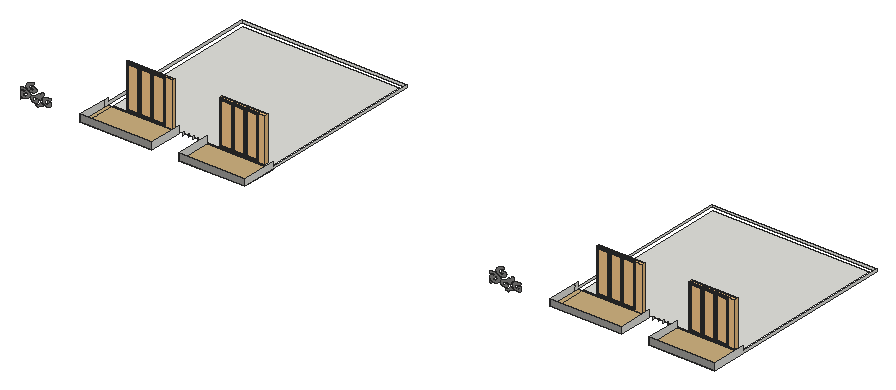
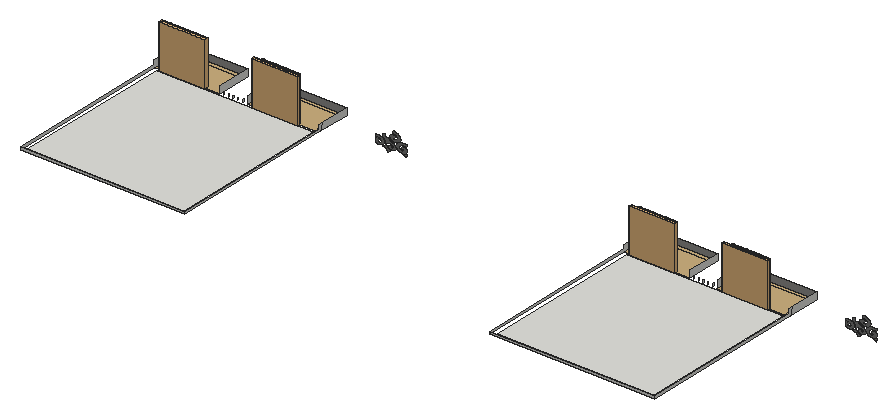
# SketchUp Ruby script. Lengths in inches.
U = 1.inch
M = Sketchup.active_model
def pt(a) = Geom::Point3d.new(a.map { |v| v * U })
def face(e, loops, mat)
  f = e.add_face(loops[0].map { |a| pt(a) })
  loops[1..].each { |l| e.add_face(l.map { |a| pt(a) }).erase! }
  f.material = f.back_material = mat if mat
  f
end
# faces: each face lists its corners as indices into pts; further lists are holes
def faces(e, pts, list, mat = nil) = list.each { |f| face(e, (f[0].is_a?(Array) ? f : [f]).map { |l| l.map { |i| pts[i] } }, mat) }
# xy, xz, yz: faces in a plane at the given z, y or x. An outline is a flat list of corners, or four numbers for a rectangle; further outlines are holes
def ring(l) = l.size == 4 ? [[l[0], l[1]], [l[2], l[1]], [l[2], l[3]], [l[0], l[3]]] : l.each_slice(2).to_a
def flat(e, list, mat, &to3) = list.each { |f| face(e, (f[0].is_a?(Array) ? f : [f]).map { |l| ring(l).map { |u, v| to3.(u, v) } }, mat) }
def xy(e, z, list, mat = nil) = flat(e, list, mat) { |x, y| [x, y, z] }
def xz(e, y, list, mat = nil) = flat(e, list, mat) { |x, z| [x, y, z] }
def yz(e, x, list, mat = nil) = flat(e, list, mat) { |y, z| [x, y, z] }
def lines(e, pts, list) = list.each { |a, b| e.add_line(pt(pts[a]), pt(pts[b])) }
# prism: a flat outline (further loops are holes) pulled along v
def prism(e, loops, v, mat = nil)
  f = face(e, loops, mat); d = Geom::Vector3d.new(v.map { |x| x * U })
  f.pushpull(f.normal.samedirection?(d) ? d.length : -d.length)
end
def box(e, o, s, mat = nil) = prism(e, [[o, [o[0] + s[0], o[1], o[2]], [o[0] + s[0], o[1] + s[1], o[2]], [o[0], o[1] + s[1], o[2]]]], [0, 0, s[2]], mat)
def at(x, y, z, deg = 0) = Geom::Transformation.translation(pt([x, y, z])) * Geom::Transformation.rotation(ORIGIN, Z_AXIS, deg.degrees)
def axes(o, x, y, z) = Geom::Transformation.new([*x, 0, *y, 0, *z, 0, *pt(o).to_a, 1])
def part(name) = M.definitions.add(name)
# library, detail: a bought-in or finely detailed component or shape, given as its bounding box
def library(name, o, s) = part(name).tap { |d| box(d.entities, o, s) }
def detail(e, o, s) = box(e.add_group.entities, o, s)
def put(e, d, t, mat = nil) = e.add_instance(d, t).tap { |i| i.material = mat if mat }
def group(e, t, mat = nil) = e.add_group.tap { |g| g.transformation = t; g.material = mat if mat }.entities
root = M.entities
M.materials.add("Wine2").color = [0, 0, 0]
M.materials["Wine2"].alpha = 0
M.materials.add("[0043_SaddleBrown]4").color = [124, 123, 122]
M.materials.add("[0130_Gainsboro]").color = [39, 45, 50]
M.materials.add("[Granite Light Gray]").color = [149, 148, 144]
M.materials.add("[Wood Floor Light]").color = [204, 176, 127]
c1 = part("Framed glazing panel")
xy(c1.entities,0,[[0,-0.98,43.07,0],[0,0,43.07,1.4]],"[0130_Gainsboro]")
xy(c1.entities,0.3,[[0.3,-1.43,42.77,-0.98]],"[0130_Gainsboro]")
xy(c1.entities,2.95,[[2.95,-1.43,40.12,-0.63],[2.95,-0.63,40.12,0],[2.95,0,40.12,0.64],[2.95,0.64,40.12,1.4]],"[0130_Gainsboro]")
xy(c1.entities,3.54,[[3.54,-0.63,39.53,0],[3.54,0,39.53,0.64]],"[0130_Gainsboro]")
xy(c1.entities,111.8125,[[3.54,-0.63,39.53,0],[3.54,0,39.53,0.64]],"[0130_Gainsboro]")
xy(c1.entities,112.4,[[2.95,-1.43,40.12,-0.63],[2.95,-0.63,40.12,0],[2.95,0,40.12,0.64],[2.95,0.64,40.12,1.4]],"[0130_Gainsboro]")
xy(c1.entities,115.05,[[0.3,-1.43,42.77,-0.98]],"[0130_Gainsboro]")
xy(c1.entities,115.35,[[0,-0.98,43.07,0],[0,0,43.07,1.4]],"[0130_Gainsboro]")
xz(c1.entities,-1.43,[[[0.3,0.3,42.77,115.05],[2.95,2.95,40.12,112.4]]],"[0130_Gainsboro]")
xz(c1.entities,-0.98,[[[0,0,43.07,115.35],[0.3,0.3,42.77,115.05]]],"[0130_Gainsboro]")
xz(c1.entities,-0.63,[[[2.95,2.95,40.12,112.4],[3.54,3.54,39.53,111.8125]]],"[0130_Gainsboro]")
xz(c1.entities,0,[[3.54,3.54,39.53,111.8125]],"Wine2")
xz(c1.entities,0,[[[0,0,43.07,115.35],[2.95,2.95,40.12,112.4]],[[2.95,2.95,40.12,112.4],[3.54,3.54,39.53,111.8125]]],"[0130_Gainsboro]")
xz(c1.entities,0.64,[[[2.95,2.95,40.12,112.4],[3.54,3.54,39.53,111.8125]]],"[0130_Gainsboro]")
xz(c1.entities,1.4,[[[0,0,43.07,115.35],[2.95,2.95,40.12,112.4]]],"[0130_Gainsboro]")
yz(c1.entities,0,[[-0.98,0,0,115.35],[0,0,1.4,115.35]],"[0130_Gainsboro]")
yz(c1.entities,0.3,[[-1.43,0.3,-0.98,115.05]],"[0130_Gainsboro]")
yz(c1.entities,2.95,[[-1.43,2.95,-0.63,112.4],[-0.63,2.95,0,112.4],[0,2.95,0.64,112.4],[0.64,2.95,1.4,112.4]],"[0130_Gainsboro]")
yz(c1.entities,3.54,[[-0.63,3.54,0,111.8125],[0,3.54,0.64,111.8125]],"[0130_Gainsboro]")
yz(c1.entities,39.53,[[-0.63,3.54,0,111.8125],[0,3.54,0.64,111.8125]],"[0130_Gainsboro]")
yz(c1.entities,40.12,[[-1.43,2.95,-0.63,112.4],[-0.63,2.95,0,112.4],[0,2.95,0.64,112.4],[0.64,2.95,1.4,112.4]],"[0130_Gainsboro]")
yz(c1.entities,42.77,[[-1.43,0.3,-0.98,115.05]],"[0130_Gainsboro]")
yz(c1.entities,43.07,[[-0.98,0,0,115.35],[0,0,1.4,115.35]],"[0130_Gainsboro]")
c2 = part("Glazing assembly")
put(c2.entities,c1,axes([90.57,1.43,0],[1.05148,0,0],[0,1,0],[0,0,1]))
put(c2.entities,c1,axes([0,1.43,0],[1.05148,0,0],[0,1,0],[0,0,1]))
put(c2.entities,c1,axes([45.29,1.43,0],[1.05148,0,0],[0,1,0],[0,0,1]))
c3 = library("Curtains",[0,0,0],[121.73,8.19,117.22])
xy(root,514.875,[[3103.26,651.03,3204.51,657.03],[3351.01,651.03,3452.26,657.03],[4353.89,651.03,4455.14,657.03],[4601.63,651.03,4702.88,657.03]])
xy(root,520.4375,[[3064.33,657.03,3480.11,1085.17],[4314.96,657.03,4730.74,1085.17]])
xy(root,520.4375,[[3053.01,559.875,3243.69,570.83],[3316.14,559.875,3491.44,570.83],[4303.63,559.875,4494.32,570.83],[4566.77,559.875,4742.06,570.83],[3053.01,570.83,3064.33,651.03],
  [3064.33,570.83,3243.69,651.03],[3316.14,570.83,3480.11,651.03],[3480.11,570.83,3491.44,651.03],[4303.63,570.83,4314.96,651.03],[4314.96,570.83,4494.32,651.03],
  [4566.77,570.83,4730.74,651.03],[4730.74,570.83,4742.06,651.03]],"[Wood Floor Light]")
xz(root,559.875,[[3053.01,520.4375,3243.69,538.1875],[3316.14,520.4375,3491.44,538.1875],[4303.63,520.4375,4494.32,538.1875],[4566.77,520.4375,4742.06,538.1875]],"[Granite Light Gray]")
xz(root,589.17,[[2918.13,494.52,2917.65,494.86,2917.14,495.2,2916.62,495.53,2916.08,495.84,2915.52,496.14,2914.94,496.43,2914.34,496.71,2913.73,496.97,2913.11,497.21,2912.47,497.45,2911.81,497.67,2911.14,497.87,2912.71,498.36,2914.21,498.91,2915.64,499.53,2917,500.21,2918.28,500.95,2919.47,501.74,2920.5625,502.59,2921.55,503.48,2922.44,504.4,2923.22,505.37,2923.88,506.37,2924.43,507.39,2924.98,507,2925.54,506.61,2926.11,506.23,2926.69,505.86,2927.29,505.49,2927.89,505.13,2928.5,504.77,2929.12,504.42,2930.38,503.74,2931.03,503.41,2931.6875,503.08,2930.03,502.8125,2928.42,502.44,2926.875,501.98,2925.41,501.42,2924.05,500.78,2922.79,500.0625,2921.65,499.27,2920.65,498.42,2919.79,497.5,2919.08,496.54,2918.52,495.54],[4168.75,494.52,4168.27,494.86,4167.77,495.2,4167.25,495.53,4166.7,495.84,4166.14,496.14,4165.56,496.43,4164.97,496.71,4164.36,496.97,4163.73,497.21,4163.09,497.45,4162.44,497.67,4161.77,497.87,4163.33,498.36,4164.83,498.91,4166.27,499.53,4167.63,500.21,4168.91,500.95,4170.09,501.74,4171.1875,502.59,4172.18,503.48,4173.07,504.4,4173.84,505.37,4174.51,506.37,4175.05,507.39,4175.6,507,4176.17,506.61,4176.74,506.23,4177.32,505.86,4177.91,505.49,4178.51,505.13,4179.12,504.77,4179.74,504.42,4180.37,504.08,4181.01,503.74,4181.66,503.41,4182.3125,503.08,4180.65,502.8125,4179.04,502.44,4177.5,501.98,4176.04,501.42,4174.67,500.78,4173.41,500.0625,4172.28,499.27,4171.28,498.42,4170.41,497.5,4169.7,496.54,4169.15,495.54],[2869.93,499.68,2869.93,504.25,2870.35,503.96,2870.79,503.69,2871.24,503.43,2871.71,503.18,2872.21,502.95,2872.71,502.73,2873.24,502.52,2873.77,502.32,2874.89,501.98,2875.46,501.83,2876.05,501.7,2875.67,501.42,2875.26,501.16,2874.82,500.91,2874.35,500.68,2873.86,500.48,2873.34,500.29,2872.81,500.13,2872.26,499.99,2871.6875,499.875,2871.11,499.78,2870.53,499.72],[4120.56,499.68,4120.56,504.25,4120.97,503.96,4121.41,503.69,4121.87,503.43,4122.34,503.18,4122.83,502.95,4123.34,502.73,4123.86,502.52,4124.4,502.32,4124.95,502.15,4125.51,501.98,4126.09,501.83,4126.67,501.7,4126.29,501.42,4125.88,501.16,4125.44,500.91,4124.97,500.68,4124.48,500.48,4123.97,500.29,4123.43,500.13,4122.88,499.99,4122.3125,499.875,4121.74,499.78,4121.15,499.72],[2907.36,502.53,2905.92,502.63,2904.53,502.875,2903.22,503.24,2902.01,503.73,2900.9375,504.32,2900.02,505.01,2899.29,505.77,2898.75,506.59,2898.42,507.46,2898.3125,508.34,2898.2,509.36,2898.26,510.38,2898.5,511.39,2898.9,512.39,2899.47,513.35,2900.2,514.27,2901.08,515.14,2902.1,515.94,2903.25,516.68,2904.52,517.34,2905.89,517.92,2907.35,518.41,2908.74,518.85,2910.08,519.35,2911.35,519.91,2912.55,520.53,2913.68,521.19,2914.74,521.91,2915.7,522.66,2916.58,523.46,2917.36,524.29,2918.04,525.16,2918.63,526.05,2919.11,526.96,2919.78,526.65,2920.52,526.39,2921.32,526.2,2922.14,526.08,2922.99,526.02,2923.84,526.04,2924.67,526.13,2925.49,526.28,2926.25,526.51,2926.97,526.79,2927.61,527.13,2928.17,527.52,2928.38,527.84,2928.53,528.17,2928.61,528.51,2928.63,528.85,2928.59,529.18,2928.49,529.52,2928.33,529.85,2928.11,530.16,2927.83,530.45,2927.5,530.73,2927.125,530.98,2926.7,531.2,2926.47,531.33,2926.29,531.48,2926.16,531.66,2926.09,531.85,2926.08,532.04,2926.125,532.23,2926.23,532.41,2926.4,532.57,2926.61,532.71,2926.86,532.83,2927.15,532.91,2927.45,532.95,2928.01,532.98,2928.57,532.95,2929.11,532.875,2929.63,532.75,2930.12,532.59,2930.57,532.38,2930.96,532.14,2931.29,531.86,2931.56,531.56,2931.75,531.24,2931.86,530.9,2931.9,530.56,2932.11,529.99,2932.26,529.41,2932.34,528.83,2932.34,528.24,2932.28,527.66,2932.15,527.08,2931.95,526.5,2931.68,525.94,2931.35,525.39,2930.95,524.86,2930.49,524.35,2929.97,523.86,2929.04,523,2928.17,522.11,2927.36,521.2,2926.625,520.27,2925.96,519.33,2925.36,518.36,2924.84,517.375,2924.39,516.38,2924.01,515.375,2923.71,514.36,2923.48,513.33,2923.33,512.3,2922.36,513.07,2921.24,513.75,2919.99,514.33,2918.62,514.8125,2917.16,515.18,2915.64,515.42,2914.08,515.55,2912.5,515.54,2910.9375,515.42,2909.42,515.16,2907.96,514.79,2906.6,514.31,2905.625,513.85,2904.76,513.32,2904.01,512.72,2903.39,512.07,2902.91,511.38,2902.58,510.65,2902.41,509.91,2902.39,509.15,2902.53,508.41,2902.83,507.67,2903.28,506.97,2903.87,506.3125,2904.41,506.0625,2905.01,505.86,2905.66,505.72,2906.33,505.64,2907.01,505.62,2907.6875,505.66,2908.35,505.77,2908.98,505.93,2909.56,506.16,2910.08,506.43,2910.53,506.74,2910.89,507.1,2910.77,507.35,2910.6875,507.61,2910.63,507.87,2910.61,508.125,2910.63,508.39,2910.68,508.65,2910.76,508.91,2910.87,509.16,2911.02,509.4,2911.19,509.64,2911.4,509.87,2911.64,510.09,2911.87,510.26,2912.14,510.4,2912.45,510.51,2912.78,510.6,2913.13,510.65,2913.49,510.67,2913.84,510.65,2914.19,510.6,2914.52,510.51,2914.83,510.4,2915.1,510.26,2915.33,510.09,2916.01,509.4,2916.48,508.65,2916.74,507.87,2916.77,507.07,2916.58,506.27,2916.17,505.51,2915.5625,504.8,2914.76,504.17,2913.8,503.63,2912.7,503.2,2911.49,502.89,2910.22,502.71,2908.8,502.55],
  [4157.98,502.53,4156.55,502.63,4155.16,502.875,4153.84,503.24,4152.64,503.73,4151.5625,504.32,4150.65,505.01,4149.91,505.77,4149.375,506.59,4149.05,507.46,4148.9375,508.34,4148.83,509.36,4148.89,510.38,4149.12,511.39,4149.53,512.39,4150.09,513.35,4150.82,514.27,4151.7,515.14,4152.72,515.94,4153.87,516.68,4155.14,517.34,4156.52,517.92,4157.98,518.41,4159.37,518.85,4160.7,519.35,4161.97,519.91,4163.18,520.53,4164.31,521.19,4165.36,521.91,4166.33,522.66,4167.2,523.46,4167.99,524.29,4168.67,525.16,4169.25,526.05,4169.73,526.96,4170.41,526.65,4171.15,526.39,4171.94,526.2,4172.77,526.08,4173.61,526.02,4174.46,526.04,4175.3,526.13,4176.11,526.28,4176.88,526.51,4177.59,526.79,4178.24,527.13,4178.8,527.52,4179,527.84,4179.15,528.17,4179.24,528.51,4179.26,528.85,4179.22,529.18,4179.12,529.52,4178.95,529.85,4178.73,530.16,4178.46,530.45,4178.125,530.73,4177.75,530.98,4177.33,531.2,4177.1,531.33,4176.91,531.48,4176.78,531.66,4176.71,531.85,4176.7,532.04,4176.75,532.23,4176.86,532.41,4177.02,532.57,4177.24,532.71,4177.49,532.83,4177.77,532.91,4178.08,532.95,4178.63,532.98,4179.19,532.95,4179.74,532.875,4180.26,532.75,4180.75,532.59,4181.19,532.38,4181.58,532.14,4181.92,531.86,4182.18,531.56,4182.37,531.24,4182.49,530.9,4182.52,530.56,4182.74,529.99,4182.88,529.41,4182.96,528.83,4182.97,528.24,4182.91,527.66,4182.77,527.08,4182.57,526.5,4182.31,525.94,4181.97,525.39,4181.58,524.86,4181.12,524.35,4180.6,523.86,4179.66,523,4178.79,522.11,4177.99,521.2,4177.25,520.27,4176.58,519.33,4175.99,518.36,4175.46,517.375,4175.01,516.38,4174.63,515.375,4174.33,514.36,4174.11,513.33,4173.95,512.3,4172.99,513.07,4171.87,513.75,4170.61,514.33,4169.24,514.8125,4167.79,515.18,4166.26,515.42,4164.7,515.55,4163.125,515.54,4161.5625,515.42,4160.04,515.16,4158.59,514.79,4157.22,514.31,4156.25,513.85,4155.38,513.32,4154.63,512.72,4154.01,512.07,4153.54,511.38,4153.21,510.65,4153.03,509.91,4153.02,509.15,4153.16,508.41,4153.45,507.67,4153.9,506.97,4154.49,506.3125,4155.04,506.0625,4155.64,505.86,4156.28,505.72,4156.95,505.64,4157.63,505.62,4158.3125,505.66,4158.97,505.77,4159.6,505.93,4160.18,506.16,4160.7,506.43,4161.15,506.74,4161.52,507.1,4161.4,507.35,4161.3125,507.61,4161.26,507.87,4161.24,508.125,4161.25,508.39,4161.3,508.65,4161.38,508.91,4161.5,509.16,4161.64,509.4,4161.82,509.64,4162.03,509.87,4162.26,510.09,4162.5,510.26,4162.77,510.4,4163.07,510.51,4163.41,510.6,4163.75,510.65,4164.11,510.67,4164.47,510.65,4164.82,510.6,4165.15,510.51,4165.45,510.4,4165.73,510.26,4165.96,510.09,4166.63,509.4,4167.1,508.65,4167.36,507.87,4167.4,507.07,4167.21,506.27,4166.8,505.51,4166.1875,504.8,4165.39,504.17,4164.42,503.63,4163.32,503.2,4162.12,502.89,4160.84,502.71,4159.42,502.55],[2880.08,503.5,2878.93,503.64,2877.79,503.84,2876.7,504.11,2875.65,504.44,2874.65,504.83,2873.72,505.28,2872.87,505.78,2872.09,506.32,2871.4,506.91,2870.8125,507.54,2870.32,508.2,2869.93,508.88,2869.93,515.77,2870.46,516.54,2871.24,517.23,2872.23,517.81,2873.38,518.25,2874.66,518.54,2876.01,518.66,2877.37,518.61,2878.6875,518.39,2879.91,518.01,2880.97,517.49,2881.84,516.85,2882.48,516.11,2882.57,515.93,2882.625,515.75,2882.63,515.56,2882.59,515.375,2882.51,515.19,2882.38,515.02,2882.22,514.87,2882.01,514.72,2881.78,514.6,2881.52,514.51,2881.24,514.43,2880.95,514.38,2880.22,514.46,2879.49,514.45,2878.76,514.36,2878.08,514.19,2877.46,513.95,2876.92,513.64,2876.49,513.27,2876.17,512.86,2875.99,512.42,2875.93,511.97,2876.01,511.52,2876.23,511.09,2876.41,510.53,2876.74,509.99,2877.19,509.49,2877.77,509.04,2878.46,508.65,2879.24,508.34,2880.09,508.1,2880.99,507.95,2881.92,507.89,2882.85,507.91,2883.76,508.03,2884.64,508.24,2885.99,508.91,2887.18,509.6875,2888.18,510.5625,2888.96,511.52,2889.52,512.53,2889.84,513.58,2889.91,514.65,2889.74,515.71,2889.32,516.75,2888.67,517.74,2887.79,518.67,2886.72,519.51,2886.28,520.06,2885.76,520.6,2885.18,521.1,2884.53,521.57,2883.82,522.01,2883.06,522.41,2882.24,522.77,2881.37,523.08,2880.47,523.35,2879.53,523.58,2878.57,523.75,2877.58,523.875,2876.88,523.93,2876.17,523.94,2875.47,523.92,2874.77,523.86,2874.08,523.77,2873.4,523.64,2872.75,523.48,2872.12,523.28,2871.52,523.05,2870.95,522.8,2870.42,522.51,2869.93,522.2,2869.93,526.94,2872.08,527.38,2874.29,527.66,2876.55,527.78,2878.81,527.72,2881.04,527.51,2883.22,527.125,2885.3,526.59,2887.27,525.9,2889.09,525.07,2890.73,524.12,2892.18,523.05,2893.41,521.88,2895.07,520.15,2896.23,518.26,2896.84,516.28,2896.89,514.26,2896.37,512.26,2895.3,510.36,2893.7,508.59,2891.64,507.02,2889.17,505.69,2886.36,504.64,2883.3,503.91],[4130.71,503.5,4129.55,503.64,4128.42,503.84,4127.32,504.11,4126.27,504.44,4125.28,504.83,4124.35,505.28,4123.49,505.78,4122.72,506.32,4122.03,506.91,4121.4375,507.54,4120.95,508.2,4120.56,508.88,4120.56,515.77,4121.09,516.54,4121.86,517.23,4122.85,517.81,4124.01,518.25,4125.29,518.54,4126.64,518.66,4128,518.61,4129.3125,518.39,4130.53,518.01,4131.6,517.49,4132.47,516.85,4133.11,516.11,4133.2,515.93,4133.25,515.75,4133.25,515.56,4133.22,515.375,4133.13,515.19,4133.01,515.02,4132.84,514.87,4132.64,514.72,4132.41,514.6,4132.15,514.51,4131.87,514.43,4131.57,514.38,4130.85,514.46,4130.11,514.45,4129.39,514.36,4128.71,514.19,4128.09,513.95,4127.55,513.64,4127.12,513.27,4126.8,512.86,4126.61,512.42,4126.56,511.97,4126.64,511.52,4126.85,511.09,4127.04,510.53,4127.36,509.99,4127.82,509.49,4128.4,509.04,4129.09,508.65,4129.87,508.34,4130.72,508.1,4131.62,507.95,4132.54,507.89,4133.48,507.91,4134.39,508.03,4135.26,508.24,4136.62,508.91,4137.81,509.6875,4138.8,510.5625,4139.59,511.52,4140.14,512.53,4140.46,513.58,4140.53,514.65,4140.36,515.71,4139.94,516.75,4139.29,517.74,4138.42,518.67,4137.34,519.51,4136.9,520.06,4136.39,520.6,4135.81,521.1,4135.16,521.57,4134.45,522.01,4133.68,522.41,4132.86,522.77,4132,523.08,4131.09,523.35,4130.16,523.58,4129.19,523.75,4128.21,523.875,4127.5,523.93,4126.8,523.94,4126.09,523.92,4125.39,523.86,4124.7,523.77,4124.03,523.64,4123.375,523.48,4122.74,523.28,4122.14,523.05,4121.58,522.8,4121.05,522.51,4120.56,522.2,4120.56,526.94,4122.7,527.38,4124.92,527.66,4127.17,527.78,4129.43,527.72,4131.67,527.51,4133.84,527.125,4135.93,526.59,4137.89,525.9,4139.71,525.07,4141.36,524.12,4142.8,523.05,4144.03,521.88,4145.7,520.15,4146.86,518.26,4147.47,516.28,4147.51,514.26,4146.99,512.26,4145.92,510.36,4144.33,508.59,4142.27,507.02,4139.8,505.69,4136.99,504.64,4133.93,503.91],[2942.88,504.03,2941.53,504.08,2940.19,504.23,2938.9,504.49,2937.66,504.83,2936.5,505.27,2935.44,505.79,2934.55,506.32,2933.72,506.89,2932.94,507.49,2932.24,508.12,2931.61,508.78,2931.05,509.46,2930.57,510.16,2930.16,510.89,2929.83,511.625,2929.59,512.37,2929.43,513.13,2929.35,513.89,2929.46,515.5,2929.97,517.08,2930.86,518.59,2932.11,520.01,2933.69,521.29,2935.57,522.41,2937.7,523.35,2940.04,524.07,2942.52,524.58,2945.11,524.85,2947.73,524.875,2950.32,524.66,2950.32,520.65,2948.09,520.7,2945.88,520.51,2943.76,520.08,2941.79,519.43,2940.04,518.59,2938.55,517.57,2937.37,516.41,2936.54,515.13,2936.08,513.79,2936.01,512.42,2936.32,511.07,2937.02,509.76,2937.8125,509.21,2938.77,508.75,2939.84,508.42,2941,508.21,2942.2,508.14,2943.4,508.21,2944.56,508.42,2945.63,508.76,2946.58,509.22,2947.375,509.78,2947.98,510.42,2948.38,511.12,2948.46,511.4,2948.45,511.6875,2948.36,511.97,2948.2,512.24,2947.96,512.49,2947.66,512.71,2947.3,512.89,2946.9,513.03,2946.46,513.13,2946,513.1875,2945.53,513.1875,2945.07,513.14,2944.82,513.21,2944.6,513.29,2944.38,513.39,2944.1875,513.5,2944.01,513.62,2943.86,513.75,2943.73,513.89,2943.63,514.04,2943.55,514.2,2943.51,514.36,2943.49,514.52,2943.49,514.68,2943.86,515.01,2944.3,515.31,2944.8,515.57,2945.35,515.78,2945.9375,515.95,2946.56,516.07,2947.2,516.14,2947.85,516.16,2948.5,516.12,2949.14,516.03,2949.75,515.89,2950.32,515.7,2950.32,505.79,2949.26,505.27,2948.11,504.83,2946.87,504.49,2945.57,504.23,2944.24,504.08],[4193.51,504.03,4192.15,504.08,4190.82,504.23,4189.52,504.49,4188.29,504.83,4187.13,505.27,4186.07,505.79,4185.17,506.32,4184.34,506.89,4183.57,507.49,4182.87,508.12,4182.23,508.78,4181.67,509.46,4181.19,510.16,4180.79,510.89,4180.46,511.625,4180.21,512.37,4180.05,513.13,4179.97,513.89,4180.09,515.5,4180.6,517.08,4181.49,518.59,4182.74,520.01,4184.32,521.29,4186.19,522.41,4188.33,523.35,4190.66,524.07,4193.15,524.58,4195.73,524.85,4198.35,524.875,4200.95,524.66,4200.95,520.65,4198.72,520.7,4196.51,520.51,4194.39,520.08,4192.42,519.43,4190.66,518.59,4189.17,517.57,4188,516.41,4187.16,515.13,4186.7,513.79,4186.63,512.42,4186.95,511.07,4187.64,509.76,4188.4375,509.21,4189.39,508.75,4190.47,508.42,4191.625,508.21,4192.83,508.14,4194.03,508.21,4195.19,508.42,4196.26,508.76,4197.21,509.22,4198,509.78,4198.61,510.42,4199.01,511.12,4199.08,511.4,4199.07,511.6875,4198.99,511.97,4198.82,512.24,4198.59,512.49,4198.28,512.71,4197.93,512.89,4197.52,513.03,4197.08,513.13,4196.62,513.1875,4196.15,513.1875,4195.69,513.14,4195.45,513.21,4195.22,513.29,4195.01,513.39,4194.8125,513.5,4194.64,513.62,4194.49,513.75,4194.36,513.89,4194.26,514.04,4194.18,514.2,4194.13,514.36,4194.11,514.52,4194.12,514.68,4194.49,515.01,4194.92,515.31,4195.42,515.57,4195.97,515.78,4196.5625,515.95,4197.18,516.07,4197.82,516.14,4198.48,516.16,4199.125,516.12,4199.76,516.03,4200.37,515.89,4200.95,515.7,4200.95,505.79,4199.89,505.27,4198.73,504.83,4197.49,504.49,4196.2,504.23,4194.86,504.08],
  [2900.77,524.15,2898.4375,524.23,2896.15,524.54,2893.97,525.06,2891.95,525.78,2890.14,526.69,2888.59,527.76,2887.32,528.97,2886.375,530.28,2885.77,531.67,2885.54,533.1,2885.66,534.54,2886.15,535.94,2886.71,537.31,2887.46,538.63,2888.42,539.91,2889.56,541.13,2890.87,542.28,2892.35,543.35,2893.99,544.33,2895.77,545.22,2897.67,546,2899.68,546.68,2901.78,547.23,2903.96,547.67,2904.37,547.29,2904.73,546.89,2905.05,546.47,2905.31,546.05,2905.52,545.61,2905.67,545.16,2905.78,544.71,2905.82,544.26,2905.81,543.8,2905.74,543.35,2905.625,542.9,2905.45,542.45,2904.1,542.55,2902.74,542.53,2901.39,542.4,2900.09,542.15,2898.86,541.8,2897.72,541.34,2896.6875,540.79,2895.79,540.17,2895.05,539.47,2894.46,538.71,2894.06,537.91,2893.83,537.09,2893.47,536.31,2893.24,535.51,2893.15,534.7,2893.2,533.89,2893.39,533.09,2893.72,532.31,2894.19,531.55,2894.79,530.82,2895.5,530.14,2896.34,529.51,2897.28,528.94,2898.31,528.4375,2899.26,528.1,2900.31,527.875,2901.4,527.78,2902.51,527.81,2903.58,527.97,2904.59,528.25,2905.49,528.64,2906.26,529.13,2906.86,529.7,2907.27,530.33,2907.49,531,2907.49,531.68,2907.4,532.01,2907.24,532.34,2907.01,532.64,2906.72,532.93,2906.36,533.1875,2905.95,533.41,2905.49,533.6,2904.99,533.75,2904.47,533.86,2903.93,533.92,2903.375,533.9375,2902.83,533.91,2902.25,533.89,2901.6875,533.96,2901.16,534.1,2900.7,534.3125,2900.34,534.58,2900.08,534.9,2899.94,535.24,2899.9375,535.59,2900.0625,535.9375,2900.3125,536.25,2900.67,536.53,2901.125,536.75,2902.37,537.12,2903.71,537.35,2905.09,537.43,2906.48,537.35,2907.8125,537.125,2909.06,536.75,2910.18,536.24,2911.12,535.61,2911.87,534.89,2912.39,534.1,2912.67,533.27,2912.69,532.41,2912.75,531.38,2912.57,530.35,2912.17,529.35,2911.54,528.39,2910.71,527.49,2909.68,526.68,2908.48,525.95,2907.13,525.33,2905.66,524.84,2904.09,524.47,2902.45,524.24],[4151.4,524.15,4149.0625,524.23,4146.78,524.54,4144.6,525.06,4142.58,525.78,4140.77,526.69,4139.21,527.76,4137.94,528.97,4137,530.28,4136.4,531.67,4136.16,533.1,4136.29,534.54,4136.78,535.94,4137.33,537.31,4138.09,538.63,4139.04,539.91,4140.18,541.13,4141.5,542.28,4142.98,543.35,4144.62,544.33,4146.39,545.22,4148.29,546,4150.3,546.68,4152.41,547.23,4154.58,547.67,4154.99,547.29,4155.36,546.89,4155.67,546.47,4155.93,546.05,4156.14,545.61,4156.3,545.16,4156.4,544.71,4156.45,544.26,4156.44,543.8,4156.37,543.35,4156.25,542.9,4156.07,542.45,4154.72,542.55,4153.36,542.53,4152.02,542.4,4150.72,542.15,4149.48,541.8,4148.34,541.34,4147.3125,540.79,4146.42,540.17,4145.67,539.47,4145.09,538.71,4144.68,537.91,4144.46,537.09,4144.09,536.31,4143.86,535.51,4143.77,534.7,4143.82,533.89,4144.02,533.09,4144.35,532.31,4144.81,531.55,4145.41,530.82,4146.13,530.14,4146.96,529.51,4147.9,528.94,4148.93,528.4375,4149.89,528.1,4150.93,527.875,4152.03,527.78,4153.13,527.81,4154.21,527.97,4155.22,528.25,4156.12,528.64,4156.88,529.13,4157.49,529.7,4157.9,530.33,4158.11,531,4158.12,531.68,4158.03,532.01,4157.87,532.34,4157.64,532.64,4157.34,532.93,4156.98,533.1875,4156.57,533.41,4156.11,533.6,4155.62,533.75,4155.1,533.86,4154.55,533.92,4154,533.9375,4153.45,533.91,4152.88,533.89,4152.3125,533.96,4151.79,534.1,4151.33,534.3125,4150.96,534.58,4150.7,534.9,4150.57,535.24,4150.5625,535.59,4150.6875,535.9375,4150.9375,536.25,4151.3,536.53,4151.75,536.75,4153,537.12,4154.33,537.35,4155.72,537.43,4157.1,537.35,4158.4375,537.125,4159.69,536.75,4160.8,536.24,4161.75,535.61,4162.49,534.89,4163.01,534.1,4163.29,533.27,4163.32,532.41,4163.37,531.38,4163.2,530.35,4162.79,529.35,4162.17,528.39,4161.33,527.49,4160.31,526.68,4159.11,525.95,4157.76,525.33,4156.28,524.84,4154.71,524.47,4153.07,524.24]],"[0043_SaddleBrown]4")
xz(root,1096.5,[[3053.01,520.4375,3491.44,526.4375],[4303.63,520.4375,4742.06,526.4375]])
yz(root,3053.01,[[559.875,520.4375,640.11,538.1875],[640.11,520.4375,640.11,538.1875,651.03,538.1875,651.03,526.4375,1096.5,526.4375,1096.5,520.4375]])
yz(root,3243.69,[[559.875,520.4375,647.91,538.1875]])
yz(root,3256.69,[[647.91,520.4375,651.03,526.4375]])
yz(root,3269.44,[[648.85,520.4375,651.03,526.4375]])
yz(root,3281.57,[[648.85,520.4375,651.03,526.4375]])
yz(root,3293.94,[[648.85,520.4375,651.03,526.4375]])
yz(root,3306.82,[[648.85,520.4375,651.03,526.4375]])
yz(root,3316.14,[[559.875,520.4375,651.03,538.1875]])
yz(root,3491.44,[[559.875,520.4375,1096.5,520.4375,1096.5,526.4375,651.03,526.4375,651.03,538.1875,559.875,538.1875]])
yz(root,4303.63,[[559.875,520.4375,640.11,538.1875],[640.11,520.4375,640.11,538.1875,651.03,538.1875,651.03,526.4375,1096.5,526.4375,1096.5,520.4375]])
yz(root,4494.32,[[559.875,520.4375,647.91,538.1875]])
yz(root,4507.32,[[647.91,520.4375,651.03,526.4375]])
yz(root,4520.07,[[648.85,520.4375,651.03,526.4375]])
yz(root,4532.19,[[648.85,520.4375,651.03,526.4375]])
yz(root,4544.57,[[648.85,520.4375,651.03,526.4375]])
yz(root,4557.44,[[648.85,520.4375,651.03,526.4375]])
yz(root,4566.77,[[559.875,520.4375,651.03,538.1875]])
yz(root,4742.06,[[559.875,520.4375,1096.5,520.4375,1096.5,526.4375,651.03,526.4375,651.03,538.1875,559.875,538.1875]])
p = [[2869.93,589.17,496.56],[2869.93,589.17,499.68],[4120.56,589.17,496.56],[4120.56,589.17,499.68]]
lines(root,p,[[0,1],[2,3]])
put(root,c2,axes([3102.86,650.7,523.79],[0.75,0,0],[0,0.75,0],[0,0,1.01765]))
put(root,c3,at(3103.29,651.77,521.91))
put(root,c2,axes([3350.36,651.03,523.48],[0.75,0,0],[0,0.75,0],[0,0,1.01765]))
put(root,c3,at(3349.11,652.22,523.95))
put(root,c2,axes([4353.48,650.7,523.79],[0.75,0,0],[0,0.75,0],[0,0,1.01765]))
put(root,c3,at(4353.91,651.77,521.91))
put(root,c2,axes([4600.98,651.03,523.48],[0.75,0,0],[0,0.75,0],[0,0,1.01765]))
put(root,c3,at(4599.74,652.22,523.95))
